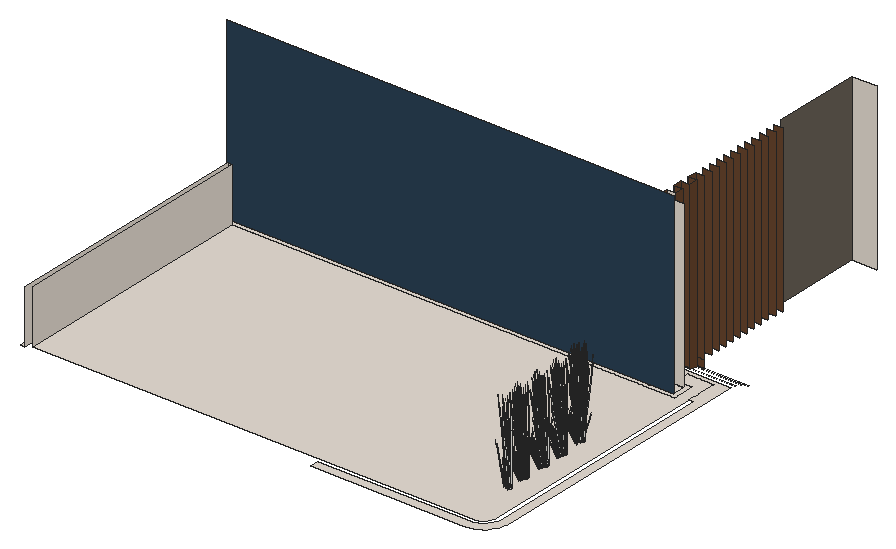
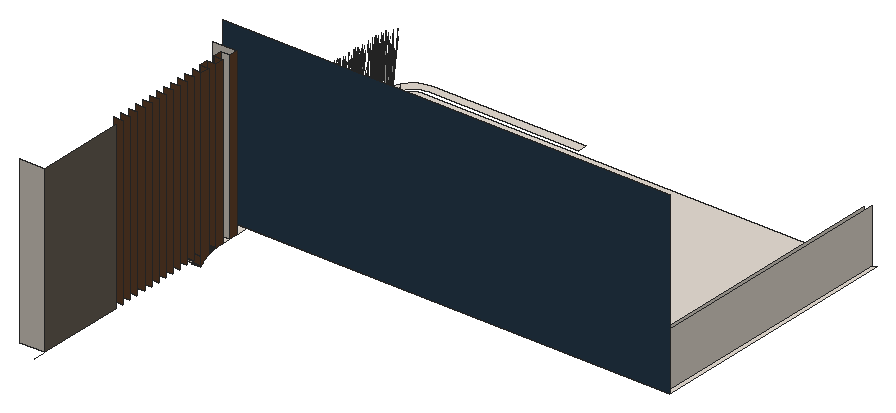
# SketchUp Ruby script. Lengths in inches.
U = 1.inch
M = Sketchup.active_model
def pt(a) = Geom::Point3d.new(a.map { |v| v * U })
def face(e, loops, mat)
  f = e.add_face(loops[0].map { |a| pt(a) })
  loops[1..].each { |l| e.add_face(l.map { |a| pt(a) }).erase! }
  f.material = f.back_material = mat if mat
  f
end
# faces: each face lists its corners as indices into pts; further lists are holes
def faces(e, pts, list, mat = nil) = list.each { |f| face(e, (f[0].is_a?(Array) ? f : [f]).map { |l| l.map { |i| pts[i] } }, mat) }
# xy, xz, yz: faces in a plane at the given z, y or x. An outline is a flat list of corners, or four numbers for a rectangle; further outlines are holes
def ring(l) = l.size == 4 ? [[l[0], l[1]], [l[2], l[1]], [l[2], l[3]], [l[0], l[3]]] : l.each_slice(2).to_a
def flat(e, list, mat, &to3) = list.each { |f| face(e, (f[0].is_a?(Array) ? f : [f]).map { |l| ring(l).map { |u, v| to3.(u, v) } }, mat) }
def xy(e, z, list, mat = nil) = flat(e, list, mat) { |x, y| [x, y, z] }
def xz(e, y, list, mat = nil) = flat(e, list, mat) { |x, z| [x, y, z] }
def yz(e, x, list, mat = nil) = flat(e, list, mat) { |y, z| [x, y, z] }
def lines(e, pts, list) = list.each { |a, b| e.add_line(pt(pts[a]), pt(pts[b])) }
# prism: a flat outline (further loops are holes) pulled along v
def prism(e, loops, v, mat = nil)
  f = face(e, loops, mat); d = Geom::Vector3d.new(v.map { |x| x * U })
  f.pushpull(f.normal.samedirection?(d) ? d.length : -d.length)
end
def box(e, o, s, mat = nil) = prism(e, [[o, [o[0] + s[0], o[1], o[2]], [o[0] + s[0], o[1] + s[1], o[2]], [o[0], o[1] + s[1], o[2]]]], [0, 0, s[2]], mat)
def at(x, y, z, deg = 0) = Geom::Transformation.translation(pt([x, y, z])) * Geom::Transformation.rotation(ORIGIN, Z_AXIS, deg.degrees)
def axes(o, x, y, z) = Geom::Transformation.new([*x, 0, *y, 0, *z, 0, *pt(o).to_a, 1])
def part(name) = M.definitions.add(name)
# library, detail: a bought-in or finely detailed component or shape, given as its bounding box
def library(name, o, s) = part(name).tap { |d| box(d.entities, o, s) }
def detail(e, o, s) = box(e.add_group.entities, o, s)
def put(e, d, t, mat = nil) = e.add_instance(d, t).tap { |i| i.material = mat if mat }
def group(e, t, mat = nil) = e.add_group.tap { |g| g.transformation = t; g.material = mat if mat }.entities
root = M.entities
M.materials.add("Carpet_04_1K").color = [43, 65, 85]
M.materials.add("LightPink_Translucent").color = [144, 107, 117]
M.materials["LightPink_Translucent"].alpha = 0.75
M.materials.add("Marble_01_1K").color = [230, 221, 211]
M.materials.add("Plaster_04_1K").color = [106, 98, 87]
M.materials.add("Wood_Veneer_15_1K").color = [103, 69, 45]
c1 = part("blade")
p = [[2.15,0.21,22],[0,0.17,0],[0.09,0.45,0],[2.18,0.31,22],[2.29,0.31,22],[0.38,0.45,0],
  [2.48,0.24,33],[2.49,0.24,33],[2.48,0.22,33]]
faces(c1.entities,p,[[0,1,2,3],[4,5,2,3],[6,3,4,7],[8,0,3,6]])
c2 = part("seeds")
p = [[0.3,-0.1,1.38],[-0.01,-0.03,1.59],[-0.01,-0.03,0.03],[0.14,-0.07,-0.07],[0.29,-0.03,3],[0.15,0.01,3.11]]
faces(c2.entities,p,[[0,1,2,3],[1,0,4,5]],"LightPink_Translucent")
c3 = part("blade with seeds")
put(c3.entities,c1,at(0,0,0))
put(c3.entities,c2,axes([2.4,0.25,30.99],[1.5799,-0.05474,1.17369],[-0.12525,1.92788,0.29478],[-0.07173,-0.02425,1.56792]))
xy(root,264,[[237,36,339,36,341.38,36.08,343.72,36.47,345.99,37.19,348.14,38.21,350.13,39.51,351.92,41.08,353.49,42.87,354.79,44.86,355.81,47.01,356.53,49.28,356.92,51.62,357,54,357,240,321,240,321,237,327,237,327,231,321,231,321,225,337.5,225,337.5,216,39,216,39,213,340.5,213,340.5,228,330,228,330,237,348,237,348,216,351,216,351,54,350.875,52.44,350.55,50.91,350.03,49.44,349.33,48.04,348.46,46.75,347.42,45.58,346.25,44.54,344.96,43.67,343.56,42.97,342.09,42.45,340.56,42.125,339,42,237,42],[36,42,39,216],[42,45,338.95,45,340.125,45.1,341.28,45.34,342.39,45.73,343.44,46.26,344.42,46.92,345.3,47.7,346.08,48.58,346.74,49.56,347.27,50.61,347.66,51.72,347.9,52.875,348,54.05,348,237,330,237,330,228,340.5,228,340.5,213,42,213],[321,216,337.5,225],[321,231,327,237]],"Marble_01_1K")
xz(root,213,[[39,264,42,300]],"Marble_01_1K")
xz(root,216,[[36,264,337.5,384]],"Carpet_04_1K")
xz(root,225,[[321,264,337.5,375]],"Marble_01_1K")
xz(root,231,[[321,264,327,375]],"Marble_01_1K")
xz(root,237,[[321,264,327,375]],"Wood_Veneer_15_1K")
xz(root,243,[[321,263.74,327,264]],"Marble_01_1K")
xz(root,243,[[321,264,327,375]],"Wood_Veneer_15_1K")
xz(root,249,[[321,262.04,327,264],[321,264,327,375]],"Wood_Veneer_15_1K")
xz(root,255,[[321,258.4,327,264],[321,264,327,375]],"Wood_Veneer_15_1K")
xz(root,261,[[321,264,327,375]],"Wood_Veneer_15_1K")
xz(root,267,[[321,264,327,375]],"Wood_Veneer_15_1K")
xz(root,273,[[321,264,327,375]],"Wood_Veneer_15_1K")
xz(root,279,[[321,264,327,375]],"Wood_Veneer_15_1K")
xz(root,285,[[321,264,327,375]],"Wood_Veneer_15_1K")
xz(root,291,[[321,264,327,375]],"Wood_Veneer_15_1K")
xz(root,297,[[321,264,327,375]],"Wood_Veneer_15_1K")
xz(root,303,[[321,264,327,375]],"Wood_Veneer_15_1K")
xz(root,309,[[321,264,327,375]],"Wood_Veneer_15_1K")
xz(root,315,[[321,264,327,375]],"Wood_Veneer_15_1K")
xz(root,321,[[321,264,327,375]],"Wood_Veneer_15_1K")
xz(root,387,[[321,264,337.5,375]],"Marble_01_1K")
yz(root,39,[[42,264,213,300]],"Marble_01_1K")
yz(root,42,[[45,264,213,300]],"Marble_01_1K")
yz(root,321,[[327,264,387,375]],"Plaster_04_1K")
yz(root,321,[[255,258.4,255,375,249,375,249,262.04,249.43,261.85,250.11,261.54,250.77,261.2,251.43,260.84,252.08,260.46,252.71,260.07,253.34,259.65,253.95,259.22,254.54,258.77],[242.98,263.74,243,263.74,243,375,237,375,237,264,240,264,240.75,263.97,241.49,263.91,242.24,263.84],[225,264,231,375]],"Wood_Veneer_15_1K")
yz(root,327,[[249,262.04,249,375,243,375,243,263.74,243.72,263.62,244.45,263.47,245.18,263.31,245.91,263.12,246.625,262.91,247.34,262.68,248.04,262.42,248.74,262.15],[231,264,237,375]],"Wood_Veneer_15_1K")
p = [[321,255.69,257.81],[321,255.125,258.3],[327,255.125,258.3],[327,255.69,257.81],[357,254.54,258.77],[357,255.125,258.3],
  [327,255,258.4],[321,255,258.4],[321,254.54,258.77],[357,248.74,262.15],[357,249.43,261.85],[321,249.43,261.85],
  [321,249,262.04],[327,249,262.04],[327,248.74,262.15],[321,248.74,262.15],[321,248.04,262.42],[327,248.04,262.42],
  [321,247.34,262.68],[327,247.34,262.68],[321,246.625,262.91],[327,246.625,262.91],[321,245.91,263.12],[327,245.91,263.12],
  [321,245.18,263.31],[327,245.18,263.31],[321,244.45,263.47],[327,244.45,263.47],[321,243.72,263.62],[327,243.72,263.62],
  [321,243,263.74],[327,243,263.74],[357,242.98,263.74],[357,243.72,263.62],[321,242.98,263.74],[321,387,264],
  [321,396,264]]
faces(root,p,[[0,1,2,3],[4,5,2,6,7,8],[1,7,6,2],[9,10,11,12,13,14],[12,15,14,13],[15,16,17,14],[16,18,19,17],[18,20,21,19],
  [20,22,23,21],[22,24,25,23],[24,26,27,25],[26,28,29,27],[28,30,31,29],[32,33,29,31,30,34]],"Marble_01_1K")
lines(root,p,[[35,36]])
put(root,c3,axes([330.66,143.87,266.41],[0.17773,0.04462,1.33163],[0.11455,0.45576,-0.28638],[-0.24142,0.08531,0.56934]))
put(root,c3,axes([331.35,141.67,266.41],[0.09985,0.15133,1.33163],[-0.23008,0.41134,-0.28638],[-0.23625,-0.09832,0.56934]))
put(root,c3,axes([330.99,142.68,265.39],[0.01297,0.08566,1.6421],[-0.26146,0.44735,-0.25086],[-0.18572,-0.02255,0.2797]))
put(root,c3,axes([330.85,145.08,265.39],[0.0686,0.0543,1.6421],[0.11632,0.50315,-0.25086],[-0.15204,0.10729,0.2797]))
put(root,c3,axes([332.875,125.86,266.41],[0.17773,0.04462,1.33163],[0.11455,0.45576,-0.28638],[-0.24142,0.08531,0.56934]))
put(root,c3,axes([332.875,110.02,266.41],[0.17773,0.04462,1.33163],[0.11455,0.45576,-0.28638],[-0.24142,0.08531,0.56934]))
put(root,c3,axes([332.875,93.61,266.41],[0.17773,0.04462,1.33163],[0.11455,0.45576,-0.28638],[-0.24142,0.08531,0.56934]))
put(root,c3,axes([332.875,78.72,266.41],[0.17773,0.04462,1.33163],[0.11455,0.45576,-0.28638],[-0.24142,0.08531,0.56934]))
put(root,c3,axes([332.7,143.46,265.92],[-0.53199,-0.08911,-0.58063],[0.11226,-0.54969,-0.15239],[-0.15876,-0.06661,1.28164]))
put(root,c3,axes([333.5625,123.66,266.41],[0.09985,0.15133,1.33163],[-0.23008,0.41134,-0.28638],[-0.23625,-0.09832,0.56934]))
put(root,c3,axes([333.5625,107.82,266.41],[0.09985,0.15133,1.33163],[-0.23008,0.41134,-0.28638],[-0.23625,-0.09832,0.56934]))
put(root,c3,axes([333.5625,91.4,266.41],[0.09985,0.15133,1.33163],[-0.23008,0.41134,-0.28638],[-0.23625,-0.09832,0.56934]))
put(root,c3,axes([332,144.5,265.88],[-0.47863,-0.27177,-0.46235],[0.28609,-0.48733,0],[-0.10901,-0.0619,1.46668]))
put(root,c3,axes([331.79,140.45,265.39],[-0.04954,0.0716,1.6421],[-0.50062,0.15438,-0.25086],[-0.12094,-0.14044,0.2797]))
put(root,c3,axes([332.29,144.83,266.21],[-0.31974,0.54466,0],[-0.53494,-0.30375,-0.48057],[-0.12184,-0.06918,1.52448]))
put(root,c3,axes([333.2,124.67,265.39],[0.01297,0.08566,1.6421],[-0.26146,0.44735,-0.25086],[-0.18572,-0.02255,0.2797]))
put(root,c3,axes([333.2,108.83,265.39],[0.01297,0.08566,1.6421],[-0.26146,0.44735,-0.25086],[-0.18572,-0.02255,0.2797]))
put(root,c3,axes([333.2,92.41,265.39],[0.01297,0.08566,1.6421],[-0.26146,0.44735,-0.25086],[-0.18572,-0.02255,0.2797]))
put(root,c3,axes([331.71,145.61,266.41],[0.16138,-0.08575,1.33163],[0.39845,0.25854,-0.28638],[-0.1186,0.22371,0.56934]))
put(root,c3,axes([331.48,140.73,265.98],[-0.14753,0.44383,-0.03625],[-0.45406,-0.13653,-0.16435],[-0.06894,-0.07259,0.54209]))
put(root,c3,axes([332.5,110.98,266.58],[0.21313,-0.24635,1.06958],[0.0841,0.38999,0.78586],[-0.15402,0.06983,0.23558]))
put(root,c3,axes([332.5,94.56,266.58],[0.21313,-0.24635,1.06958],[0.0841,0.38999,0.78586],[-0.15402,0.06983,0.23558]))
put(root,c3,axes([332.5,79.67,266.58],[0.21313,-0.24635,1.06958],[0.0841,0.38999,0.78586],[-0.15402,0.06983,0.23558]))
put(root,c3,axes([332.16,140.17,266.41],[-0.03097,0.17781,1.33163],[-0.45273,0.14885,-0.28638],[-0.10583,-0.22982,0.56934]))
put(root,c3,axes([333.3,143.54,266.48],[-0.51635,0.36087,-0.27094],[-0.34336,-0.5099,-0.46562],[-0.1274,-0.05178,1.4872]))
put(root,c3,axes([331.24,142.75,266.21],[-0.63949,0,0],[0,-0.60749,-0.48057],[0,-0.13836,1.52448]))
put(root,c3,axes([332.13,144.3,265.89],[-0.12013,-0.47362,-0.28847],[0.47712,-0.13449,0.28847],[-0.09619,-0.05462,1.29413]))
put(root,c3,axes([333.06,127.07,265.39],[0.0686,0.0543,1.6421],[0.11632,0.50315,-0.25086],[-0.15204,0.10729,0.2797]))
put(root,c3,axes([333.06,111.23,265.39],[0.0686,0.0543,1.6421],[0.11632,0.50315,-0.25086],[-0.15204,0.10729,0.2797]))
put(root,c3,axes([333.06,94.8125,265.39],[0.0686,0.0543,1.6421],[0.11632,0.50315,-0.25086],[-0.15204,0.10729,0.2797]))
put(root,c3,axes([333.06,79.93,265.39],[0.0686,0.0543,1.6421],[0.11632,0.50315,-0.25086],[-0.15204,0.10729,0.2797]))
put(root,c3,axes([332.97,124.11,266.58],[0.3265,-0.03889,1.06958],[-0.20711,0.3427,0.78586],[-0.16135,-0.05141,0.23558]))
put(root,c3,axes([332.97,108.27,266.58],[0.3265,-0.03889,1.06958],[-0.20711,0.3427,0.78586],[-0.16135,-0.05141,0.23558]))
put(root,c3,axes([332.97,91.85,266.58],[0.3265,-0.03889,1.06958],[-0.20711,0.3427,0.78586],[-0.16135,-0.05141,0.23558]))
put(root,c3,axes([333.65,143.93,265.92],[-0.34446,0.40855,-0.58063],[-0.42791,-0.37046,-0.15239],[-0.13803,0.10191,1.28164]))
put(root,c3,axes([331.73,142.59,266.17],[-0.47569,0.45698,0.2864],[-0.47598,-0.45217,-0.33981],[-0.01661,-0.12977,1.53541]))
put(root,c3,axes([333.88,143.7,266.3],[-0.49938,-0.43748,-0.23459],[0.42021,-0.49126,0.51337],[-0.13447,0.05118,1.56642]))
put(root,c3,axes([332.98,143.28,266.06],[-0.30722,-0.45622,-0.41661],[0.46535,-0.32126,0.2005],[-0.09942,-0.05645,1.33761]))
put(root,c3,axes([333.63,143.61,266.06],[-0.55535,0.03355,-0.41661],[-0.05022,-0.55698,0.2005],[-0.09942,0.05645,1.33761]))
put(root,c3,axes([332.57,144.54,266.31],[0.47863,0.27177,0.46235],[-0.28609,0.48733,0],[-0.10901,-0.0619,1.46668]))
put(root,c3,axes([334.91,125.45,265.92],[-0.53199,-0.08911,-0.58063],[0.11226,-0.54969,-0.15239],[-0.15876,-0.06661,1.28164]))
put(root,c3,axes([334.91,109.61,265.92],[-0.53199,-0.08911,-0.58063],[0.11226,-0.54969,-0.15239],[-0.15876,-0.06661,1.28164]))
put(root,c3,axes([334.92,93.19,265.92],[-0.53199,-0.08911,-0.58063],[0.11226,-0.54969,-0.15239],[-0.15876,-0.06661,1.28164]))
put(root,c3,axes([333.02,143.54,266.27],[0.13555,-0.64407,-0.21817],[0.64269,0.11227,0.47743],[-0.1123,-0.08895,1.45677]))
put(root,c3,axes([333.25,143.7,266.4375],[-0.09866,0.48509,0.13483],[-0.48202,-0.0842,-0.38503],[-0.08772,-0.04981,1.18024]))
put(root,c3,axes([334.21,145.05,265.88],[-0.47863,0.27177,-0.46235],[-0.28609,-0.48733,0],[-0.10901,0.0619,1.46668]))
put(root,c3,axes([331.38,142.34,265.88],[0,-0.54355,-0.46235],[0.57217,0,0],[0,-0.1238,1.46668]))
put(root,c3,axes([331.625,142.84,266.31],[0,0.54355,0.46235],[-0.57217,0,0],[0,-0.1238,1.46668]))
put(root,c3,axes([334.25,144.9,266.04],[-0.31576,-0.54657,-0.04789],[0.53494,-0.30375,0.48057],[-0.13182,0.05204,1.52373]))
put(root,c3,axes([334.22,126.49,265.88],[-0.47863,-0.27177,-0.46235],[0.28609,-0.48733,0],[-0.10901,-0.0619,1.46668]))
put(root,c3,axes([334.22,110.65,265.88],[-0.47863,-0.27177,-0.46235],[0.28609,-0.48733,0],[-0.10901,-0.0619,1.46668]))
put(root,c3,axes([334.22,94.23,265.88],[-0.47863,-0.27177,-0.46235],[0.28609,-0.48733,0],[-0.10901,-0.0619,1.46668]))
put(root,c3,axes([334.01,122.44,265.39],[-0.04954,0.0716,1.6421],[-0.50062,0.15438,-0.25086],[-0.12094,-0.14044,0.2797]))
put(root,c3,axes([334.01,106.6,265.39],[-0.04954,0.0716,1.6421],[-0.50062,0.15438,-0.25086],[-0.12094,-0.14044,0.2797]))
put(root,c3,axes([334.01,90.18,265.39],[-0.04954,0.0716,1.6421],[-0.50062,0.15438,-0.25086],[-0.12094,-0.14044,0.2797]))
put(root,c3,axes([334.1,144.83,265.89],[-0.47712,-0.13449,-0.28847],[0.12013,-0.47362,0.28847],[-0.09619,0.05462,1.29413]))
put(root,c3,axes([334.51,126.82,266.21],[-0.31974,0.54466,0],[-0.53494,-0.30375,-0.48057],[-0.12184,-0.06918,1.52448]))
put(root,c3,axes([334.51,110.98,266.21],[-0.31974,0.54466,0],[-0.53494,-0.30375,-0.48057],[-0.12184,-0.06918,1.52448]))
put(root,c3,axes([334.51,94.56,266.21],[-0.31974,0.54466,0],[-0.53494,-0.30375,-0.48057],[-0.12184,-0.06918,1.52448]))
put(root,c3,axes([334.51,79.67,266.21],[-0.31974,0.54466,0],[-0.53494,-0.30375,-0.48057],[-0.12184,-0.06918,1.52448]))
put(root,c3,axes([332.875,142.97,266.48],[-0.57594,-0.25935,-0.27094],[0.27732,-0.5474,-0.46562],[-0.0181,-0.1344,1.4872]))
put(root,c3,axes([331.82,145.2,266.63],[0.46459,-0.09625,0.0606],[0.10681,0.38778,-0.80367],[-0.02945,0.1963,0.72038]))
put(root,c3,axes([334.02,143.46,266.48],[0.05959,0.62022,-0.27094],[-0.62068,0.0375,-0.46562],[-0.1093,0.08261,1.4872]))
put(root,c3,axes([332.62,142.42,265.95],[-0.21003,-0.55738,-0.65031],[0.60499,-0.20074,-0.17068],[-0.02321,-0.18874,1.43544]))
put(root,c3,axes([333.93,127.61,266.41],[0.16138,-0.08575,1.33163],[0.39845,0.25854,-0.28638],[-0.1186,0.22371,0.56934]))
put(root,c3,axes([333.93,111.77,266.41],[0.16138,-0.08575,1.33163],[0.39845,0.25854,-0.28638],[-0.1186,0.22371,0.56934]))
put(root,c3,axes([333.93,95.35,266.41],[0.16138,-0.08575,1.33163],[0.39845,0.25854,-0.28638],[-0.1186,0.22371,0.56934]))
put(root,c3,axes([333.93,80.46,266.41],[0.16138,-0.08575,1.33163],[0.39845,0.25854,-0.28638],[-0.1186,0.22371,0.56934]))
put(root,c3,axes([333.7,122.72,265.98],[-0.14753,0.44383,-0.03625],[-0.45406,-0.13653,-0.16435],[-0.06894,-0.07259,0.54209]))
put(root,c3,axes([333.7,106.875,265.98],[-0.14753,0.44383,-0.03625],[-0.45406,-0.13653,-0.16435],[-0.06894,-0.07259,0.54209]))
put(root,c3,axes([333.7,90.46,265.98],[-0.14753,0.44383,-0.03625],[-0.45406,-0.13653,-0.16435],[-0.06894,-0.07259,0.54209]))
put(root,c3,axes([331.625,142.35,265.89],[0.35699,-0.33913,-0.28847],[0.35699,0.33913,0.28847],[0,-0.10923,1.29413]))
put(root,c3,axes([333.24,140.16,265.98],[-0.35341,0.31182,-0.03625],[-0.32382,-0.34152,-0.16435],[-0.0228,-0.09677,0.54209]))
put(root,c3,axes([333.09,143.23,266.2],[0.64638,0.11452,0.42607],[-0.13155,0.64678,0.16719],[-0.09446,-0.06245,1.47927]))
put(root,c3,axes([334.375,122.16,266.41],[-0.03097,0.17781,1.33163],[-0.45273,0.14885,-0.28638],[-0.10583,-0.22982,0.56934]))
put(root,c3,axes([334.375,106.32,266.41],[-0.03097,0.17781,1.33163],[-0.45273,0.14885,-0.28638],[-0.10583,-0.22982,0.56934]))
put(root,c3,axes([334.375,89.9,266.41],[-0.03097,0.17781,1.33163],[-0.45273,0.14885,-0.28638],[-0.10583,-0.22982,0.56934]))
put(root,c3,axes([335.52,125.53,266.48],[-0.51635,0.36087,-0.27094],[-0.34336,-0.5099,-0.46562],[-0.1274,-0.05178,1.4872]))
put(root,c3,axes([335.52,109.69,266.48],[-0.51635,0.36087,-0.27094],[-0.34336,-0.5099,-0.46562],[-0.1274,-0.05178,1.4872]))
put(root,c3,axes([335.52,93.27,266.48],[-0.51635,0.36087,-0.27094],[-0.34336,-0.5099,-0.46562],[-0.1274,-0.05178,1.4872]))
put(root,c3,axes([332.93,143.12,266.53],[-0.24813,0.48978,0.41661],[-0.51557,-0.23571,-0.2005],[0,-0.1129,1.33761]))
put(root,c3,axes([333.45,124.74,266.21],[-0.63949,0,0],[0,-0.60749,-0.48057],[0,-0.13836,1.52448]))
put(root,c3,axes([333.45,108.9,266.21],[-0.63949,0,0],[0,-0.60749,-0.48057],[0,-0.13836,1.52448]))
put(root,c3,axes([333.45,92.48,266.21],[-0.63949,0,0],[0,-0.60749,-0.48057],[0,-0.13836,1.52448]))
put(root,c3,axes([334.35,126.29,265.89],[-0.12013,-0.47362,-0.28847],[0.47712,-0.13449,0.28847],[-0.09619,-0.05462,1.29413]))
put(root,c3,axes([334.35,110.45,265.89],[-0.12013,-0.47362,-0.28847],[0.47712,-0.13449,0.28847],[-0.09619,-0.05462,1.29413]))
put(root,c3,axes([334.35,94.03,265.89],[-0.12013,-0.47362,-0.28847],[0.47712,-0.13449,0.28847],[-0.09619,-0.05462,1.29413]))
put(root,c3,axes([332.75,144.27,266.3],[0.54955,-0.14427,0.16428],[0.1357,0.53689,0.32672],[-0.04901,-0.07823,1.49371]))
put(root,c3,axes([333.45,144.35,266.05],[-0.51557,-0.24403,0],[0.24813,-0.50705,0],[0,0,1.51513]))
put(root,c3,axes([335.86,125.92,265.92],[-0.34446,0.40855,-0.58063],[-0.42791,-0.37046,-0.15239],[-0.13803,0.10191,1.28164]))
put(root,c3,axes([335.86,110.08,265.92],[-0.34446,0.40855,-0.58063],[-0.42791,-0.37046,-0.15239],[-0.13803,0.10191,1.28164]))
put(root,c3,axes([335.86,93.67,265.92],[-0.34446,0.40855,-0.58063],[-0.42791,-0.37046,-0.15239],[-0.13803,0.10191,1.28164]))
put(root,c3,axes([335.86,78.78,265.92],[-0.34446,0.40855,-0.58063],[-0.42791,-0.37046,-0.15239],[-0.13803,0.10191,1.28164]))
put(root,c3,axes([334.65,144.96,266.21],[0.31974,0.54466,0],[-0.53494,0.30375,-0.48057],[-0.12184,0.06918,1.52448]))
put(root,c3,axes([333.95,124.58,266.17],[-0.47569,0.45698,0.2864],[-0.47598,-0.45217,-0.33981],[-0.01661,-0.12977,1.53541]))
put(root,c3,axes([333.95,108.74,266.17],[-0.47569,0.45698,0.2864],[-0.47598,-0.45217,-0.33981],[-0.01661,-0.12977,1.53541]))
put(root,c3,axes([333.95,92.32,266.17],[-0.47569,0.45698,0.2864],[-0.47598,-0.45217,-0.33981],[-0.01661,-0.12977,1.53541]))
put(root,c3,axes([334.38,144.3,266.3],[0.14774,-0.54019,0.16428],[0.54062,0.15287,0.32672],[-0.09339,0.00263,1.49371]))
put(root,c3,axes([334.22,106.03,266.58],[0.26677,0.18918,1.06958],[-0.38851,0.11372,0.78586],[-0.08313,-0.14539,0.23558]))
put(root,c3,axes([334.22,89.61,266.58],[0.26677,0.18918,1.06958],[-0.38851,0.11372,0.78586],[-0.08313,-0.14539,0.23558]))
put(root,c3,axes([334.13,143.58,266.4375],[0.37783,0.32657,0.13483],[-0.31516,0.36844,-0.38503],[-0.08772,0.04981,1.18024]))
put(root,c3,axes([336.1,125.69,266.3],[-0.49938,-0.43748,-0.23459],[0.42021,-0.49126,0.51337],[-0.13447,0.05118,1.56642]))
put(root,c3,axes([336.1,109.85,266.3],[-0.49938,-0.43748,-0.23459],[0.42021,-0.49126,0.51337],[-0.13447,0.05118,1.56642]))
put(root,c3,axes([336.1,93.4375,266.3],[-0.49938,-0.43748,-0.23459],[0.42021,-0.49126,0.51337],[-0.13447,0.05118,1.56642]))
put(root,c3,axes([335.19,125.27,266.06],[-0.30722,-0.45622,-0.41661],[0.46535,-0.32126,0.2005],[-0.09942,-0.05645,1.33761]))
put(root,c3,axes([335.19,109.43,266.06],[-0.30722,-0.45622,-0.41661],[0.46535,-0.32126,0.2005],[-0.09942,-0.05645,1.33761]))
put(root,c3,axes([335.19,93.02,266.06],[-0.30722,-0.45622,-0.41661],[0.46535,-0.32126,0.2005],[-0.09942,-0.05645,1.33761]))
put(root,c3,axes([334,143.18,266.14],[-0.47569,-0.46784,-0.05709],[0.47598,-0.46812,0],[-0.01661,-0.01634,1.63492]))
put(root,c3,axes([334.125,143.34,266.53],[0.55535,-0.03355,0.41661],[0.05022,0.55698,-0.2005],[-0.09942,0.05645,1.33761]))
put(root,c3,axes([334.3125,112.05,266.58],[-0.01324,-0.32319,1.06958],[0.33072,0.23052,0.78586],[-0.06504,0.15405,0.23558]))
put(root,c3,axes([334.3125,95.63,266.58],[-0.01324,-0.32319,1.06958],[0.33072,0.23052,0.78586],[-0.06504,0.15405,0.23558]))
put(root,c3,axes([334.3125,80.75,266.58],[-0.01324,-0.32319,1.06958],[0.33072,0.23052,0.78586],[-0.06504,0.15405,0.23558]))
put(root,c3,axes([334.26,144.62,266.17],[0.64025,0.17667,0.2864],[-0.16018,0.63149,-0.33981],[-0.10597,0.07904,1.53541]))
put(root,c3,axes([335.85,125.6,266.06],[-0.55535,0.03355,-0.41661],[-0.05022,-0.55698,0.2005],[-0.09942,0.05645,1.33761]))
put(root,c3,axes([335.85,109.76,266.06],[-0.55535,0.03355,-0.41661],[-0.05022,-0.55698,0.2005],[-0.09942,0.05645,1.33761]))
put(root,c3,axes([335.85,93.34,266.06],[-0.55535,0.03355,-0.41661],[-0.05022,-0.55698,0.2005],[-0.09942,0.05645,1.33761]))
put(root,c3,axes([335.85,78.46,266.06],[-0.55535,0.03355,-0.41661],[-0.05022,-0.55698,0.2005],[-0.09942,0.05645,1.33761]))
put(root,c3,axes([333.33,139.78,265.39],[-0.08578,0.01958,1.6421],[-0.47437,-0.22044,-0.25086],[0.00796,-0.18387,0.2797]))
put(root,c3,axes([334.54,144.59,266.31],[0.47863,-0.27177,0.46235],[0.28609,0.48733,0],[-0.10901,0.0619,1.46668]))
put(root,c3,axes([333.04,142.64,266.2],[0.22235,0.6078,0.42607],[-0.63531,0.21135,0.16719],[0.00776,-0.11168,1.47927]))
put(root,c3,axes([332.9375,142.5625,266.06],[0.24813,-0.48978,-0.41661],[0.51557,0.23571,0.2005],[0,-0.1129,1.33761]))
put(root,c3,axes([333.57,144.14,266.05],[-0.16686,-0.46861,0],[0.47648,-0.16411,0],[0,0,1.4375]))
put(root,c3,axes([334.78,126.53,266.31],[0.47863,0.27177,0.46235],[-0.28609,0.48733,0],[-0.10901,-0.0619,1.46668]))
put(root,c3,axes([334.78,110.69,266.31],[0.47863,0.27177,0.46235],[-0.28609,0.48733,0],[-0.10901,-0.0619,1.46668]))
put(root,c3,axes([334.78,94.27,266.31],[0.47863,0.27177,0.46235],[-0.28609,0.48733,0],[-0.10901,-0.0619,1.46668]))
put(root,c3,axes([332.97,145.13,265.39],[0.08277,-0.02958,1.6421],[0.49786,0.16279,-0.25086],[0.01456,0.18348,0.2797]))
put(root,c3,axes([335.24,125.53,266.27],[0.13555,-0.64407,-0.21817],[0.64269,0.11227,0.47743],[-0.1123,-0.08895,1.45677]))
put(root,c3,axes([335.24,109.7,266.27],[0.13555,-0.64407,-0.21817],[0.64269,0.11227,0.47743],[-0.1123,-0.08895,1.45677]))
put(root,c3,axes([335.24,93.28,266.27],[0.13555,-0.64407,-0.21817],[0.64269,0.11227,0.47743],[-0.1123,-0.08895,1.45677]))
put(root,c3,axes([335.47,125.6875,266.4375],[-0.09866,0.48509,0.13483],[-0.48202,-0.0842,-0.38503],[-0.08772,-0.04981,1.18024]))
put(root,c3,axes([335.47,109.85,266.4375],[-0.09866,0.48509,0.13483],[-0.48202,-0.0842,-0.38503],[-0.08772,-0.04981,1.18024]))
put(root,c3,axes([335.47,93.43,266.4375],[-0.09866,0.48509,0.13483],[-0.48202,-0.0842,-0.38503],[-0.08772,-0.04981,1.18024]))
put(root,c3,axes([336.43,127.04,265.88],[-0.47863,0.27177,-0.46235],[-0.28609,-0.48733,0],[-0.10901,0.0619,1.46668]))
put(root,c3,axes([336.43,111.2,265.88],[-0.47863,0.27177,-0.46235],[-0.28609,-0.48733,0],[-0.10901,0.0619,1.46668]))
put(root,c3,axes([336.43,94.78,265.88],[-0.47863,0.27177,-0.46235],[-0.28609,-0.48733,0],[-0.10901,0.0619,1.46668]))
put(root,c3,axes([336.43,79.89,265.88],[-0.47863,0.27177,-0.46235],[-0.28609,-0.48733,0],[-0.10901,0.0619,1.46668]))
put(root,c3,axes([333.6,124.33,265.88],[0,-0.54355,-0.46235],[0.57217,0,0],[0,-0.1238,1.46668]))
put(root,c3,axes([333.6,108.49,265.88],[0,-0.54355,-0.46235],[0.57217,0,0],[0,-0.1238,1.46668]))
put(root,c3,axes([333.6,92.07,265.88],[0,-0.54355,-0.46235],[0.57217,0,0],[0,-0.1238,1.46668]))
put(root,c3,axes([333.84,124.83,266.31],[0,0.54355,0.46235],[-0.57217,0,0],[0,-0.1238,1.46668]))
put(root,c3,axes([333.84,109,266.31],[0,0.54355,0.46235],[-0.57217,0,0],[0,-0.1238,1.46668]))
put(root,c3,axes([333.84,92.58,266.31],[0,0.54355,0.46235],[-0.57217,0,0],[0,-0.1238,1.46668]))
put(root,c3,axes([336.46,126.89,266.04],[-0.31576,-0.54657,-0.04789],[0.53494,-0.30375,0.48057],[-0.13182,0.05204,1.52373]))
put(root,c3,axes([336.46,111.05,266.04],[-0.31576,-0.54657,-0.04789],[0.53494,-0.30375,0.48057],[-0.13182,0.05204,1.52373]))
put(root,c3,axes([336.46,94.63,266.04],[-0.31576,-0.54657,-0.04789],[0.53494,-0.30375,0.48057],[-0.13182,0.05204,1.52373]))
put(root,c3,axes([336.46,79.75,266.04],[-0.31576,-0.54657,-0.04789],[0.53494,-0.30375,0.48057],[-0.13182,0.05204,1.52373]))
put(root,c3,axes([334.25,143.22,266.06],[-0.24813,0.48978,-0.41661],[-0.51557,-0.23571,0.2005],[0,0.1129,1.33761]))
put(root,c3,axes([336.32,126.82,265.89],[-0.47712,-0.13449,-0.28847],[0.12013,-0.47362,0.28847],[-0.09619,0.05462,1.29413]))
put(root,c3,axes([336.32,110.98,265.89],[-0.47712,-0.13449,-0.28847],[0.12013,-0.47362,0.28847],[-0.09619,0.05462,1.29413]))
put(root,c3,axes([336.32,94.57,265.89],[-0.47712,-0.13449,-0.28847],[0.12013,-0.47362,0.28847],[-0.09619,0.05462,1.29413]))
put(root,c3,axes([336.32,79.68,265.89],[-0.47712,-0.13449,-0.28847],[0.12013,-0.47362,0.28847],[-0.09619,0.05462,1.29413]))
put(root,c3,axes([335.23,142.92,266.3],[-0.40181,-0.39593,0.16428],[0.40492,-0.38402,0.32672],[-0.04438,0.08086,1.49371]))
put(root,c3,axes([333.84,142.69,266.05],[0,-0.62892,0],[0.63949,0,0],[0,0,1.6711]))
put(root,c3,axes([335.09,124.96,266.48],[-0.57594,-0.25935,-0.27094],[0.27732,-0.5474,-0.46562],[-0.0181,-0.1344,1.4872]))
put(root,c3,axes([335.09,109.12,266.48],[-0.57594,-0.25935,-0.27094],[0.27732,-0.5474,-0.46562],[-0.0181,-0.1344,1.4872]))
put(root,c3,axes([335.09,92.7,266.48],[-0.57594,-0.25935,-0.27094],[0.27732,-0.5474,-0.46562],[-0.0181,-0.1344,1.4872]))
put(root,c3,axes([333.24,142.8,266.27],[0.57623,0.26344,0.22409],[-0.27732,0.5474,0.46562],[0,-0.12618,1.49497]))
put(root,c3,axes([334.16,142.94,266.13],[0,0.62861,-0.05249],[-0.63949,0,0],[0,0.01975,1.67027]))
put(root,c3,axes([333.06,142.4375,266.53],[-0.55535,0.03355,0.41661],[-0.05022,-0.55698,-0.2005],[0.09942,-0.05645,1.33761]))
put(root,c3,axes([332.8,141.48,266.3],[-0.14774,0.54019,0.16428],[-0.54062,-0.15287,0.32672],[0.09339,-0.00263,1.49371]))
put(root,c3,axes([333.85,144.16,266.13],[0.22235,0.62444,-0.05599],[-0.63531,0.21881,0],[0.00776,0.02181,1.60327]))
put(root,c3,axes([334.04,127.19,266.63],[0.46459,-0.09625,0.0606],[0.10681,0.38778,-0.80367],[-0.02945,0.1963,0.72038]))
put(root,c3,axes([334.04,111.35,266.63],[0.46459,-0.09625,0.0606],[0.10681,0.38778,-0.80367],[-0.02945,0.1963,0.72038]))
put(root,c3,axes([334.04,94.9375,266.63],[0.46459,-0.09625,0.0606],[0.10681,0.38778,-0.80367],[-0.02945,0.1963,0.72038]))
put(root,c3,axes([334.04,80.05,266.63],[0.46459,-0.09625,0.0606],[0.10681,0.38778,-0.80367],[-0.02945,0.1963,0.72038]))
put(root,c3,axes([336.23,125.45,266.48],[0.05959,0.62022,-0.27094],[-0.62068,0.0375,-0.46562],[-0.1093,0.08261,1.4872]))
put(root,c3,axes([336.23,109.61,266.48],[0.05959,0.62022,-0.27094],[-0.62068,0.0375,-0.46562],[-0.1093,0.08261,1.4872]))
put(root,c3,axes([336.23,93.19,266.48],[0.05959,0.62022,-0.27094],[-0.62068,0.0375,-0.46562],[-0.1093,0.08261,1.4872]))
put(root,c3,axes([336.23,78.31,266.48],[0.05959,0.62022,-0.27094],[-0.62068,0.0375,-0.46562],[-0.1093,0.08261,1.4872]))
put(root,c3,axes([334.83,124.41,265.95],[-0.21003,-0.55738,-0.65031],[0.60499,-0.20074,-0.17068],[-0.02321,-0.18874,1.43544]))
put(root,c3,axes([334.83,108.57,265.95],[-0.21003,-0.55738,-0.65031],[0.60499,-0.20074,-0.17068],[-0.02321,-0.18874,1.43544]))
put(root,c3,axes([334.83,92.15,265.95],[-0.21003,-0.55738,-0.65031],[0.60499,-0.20074,-0.17068],[-0.02321,-0.18874,1.43544]))
put(root,c3,axes([332.53,140.81,266.21],[-0.31974,-0.54466,0],[0.53494,-0.30375,-0.48057],[0.12184,-0.06918,1.52448]))
put(root,c3,axes([335.69,143.34,266.05],[-0.63917,-0.00435,-0.04634],[0,-0.60749,0.46507],[-0.02009,0.13829,1.47457]))
put(root,c3,axes([333.84,124.34,265.89],[0.35699,-0.33913,-0.28847],[0.35699,0.33913,0.28847],[0,-0.10923,1.29413]))
put(root,c3,axes([333.84,108.5,265.89],[0.35699,-0.33913,-0.28847],[0.35699,0.33913,0.28847],[0,-0.10923,1.29413]))
put(root,c3,axes([333.84,92.08,265.89],[0.35699,-0.33913,-0.28847],[0.35699,0.33913,0.28847],[0,-0.10923,1.29413]))
put(root,c3,axes([335.45,122.15,265.98],[-0.35341,0.31182,-0.03625],[-0.32382,-0.34152,-0.16435],[-0.0228,-0.09677,0.54209]))
put(root,c3,axes([335.45,106.31,265.98],[-0.35341,0.31182,-0.03625],[-0.32382,-0.34152,-0.16435],[-0.0228,-0.09677,0.54209]))
put(root,c3,axes([335.45,89.89,265.98],[-0.35341,0.31182,-0.03625],[-0.32382,-0.34152,-0.16435],[-0.0228,-0.09677,0.54209]))
put(root,c3,axes([334.43,141.51,266.3],[-0.54955,0.14427,0.16428],[-0.1357,-0.53689,0.32672],[0.04901,0.07823,1.49371]))
put(root,c3,axes([335.31,125.22,266.2],[0.64638,0.11452,0.42607],[-0.13155,0.64678,0.16719],[-0.09446,-0.06245,1.47927]))
put(root,c3,axes([335.31,109.39,266.2],[0.64638,0.11452,0.42607],[-0.13155,0.64678,0.16719],[-0.09446,-0.06245,1.47927]))
put(root,c3,axes([335.31,92.97,266.2],[0.64638,0.11452,0.42607],[-0.13155,0.64678,0.16719],[-0.09446,-0.06245,1.47927]))
put(root,c3,axes([333.54,142.29,266.2],[-0.42403,0.49328,0.42607],[-0.50377,-0.43543,0.16719],[0.10223,-0.04923,1.47927]))
put(root,c3,axes([335.14,125.11,266.53],[-0.24813,0.48978,0.41661],[-0.51557,-0.23571,-0.2005],[0,-0.1129,1.33761]))
put(root,c3,axes([335.14,109.27,266.53],[-0.24813,0.48978,0.41661],[-0.51557,-0.23571,-0.2005],[0,-0.1129,1.33761]))
put(root,c3,axes([335.14,92.85,266.53],[-0.24813,0.48978,0.41661],[-0.51557,-0.23571,-0.2005],[0,-0.1129,1.33761]))
put(root,c3,axes([334.26,143.07,266.0625],[0.35699,0.35109,0],[-0.35699,0.35109,0],[0,0,1.57621]))
put(root,c3,axes([334.26,142.66,266.53],[0.24813,-0.48978,0.41661],[0.51557,0.23571,-0.2005],[0,0.1129,1.33761]))
put(root,c3,axes([334.04,144.36,266.05],[0.51557,0.24403,0],[-0.24813,0.50705,0],[0,0,1.62917]))
put(root,c3,axes([334.09,142.54,266.22],[-0.64638,-0.11452,0.45814],[0.13155,-0.64678,0.17978],[0.09446,0.06245,1.59061]))
put(root,c3,axes([334.96,126.26,266.3],[0.54955,-0.14427,0.16428],[0.1357,0.53689,0.32672],[-0.04901,-0.07823,1.49371]))
put(root,c3,axes([334.96,110.42,266.3],[0.54955,-0.14427,0.16428],[0.1357,0.53689,0.32672],[-0.04901,-0.07823,1.49371]))
put(root,c3,axes([334.96,94,266.3],[0.54955,-0.14427,0.16428],[0.1357,0.53689,0.32672],[-0.04901,-0.07823,1.49371]))
put(root,c3,axes([335.56,143.43,265.89],[-0.35699,0.33913,-0.28847],[-0.35699,-0.33913,0.28847],[0,0.10923,1.29413]))
put(root,c3,axes([335.67,126.34,266.05],[-0.51557,-0.24403,0],[0.24813,-0.50705,0],[0,0,1.51513]))
put(root,c3,axes([335.67,110.5,266.05],[-0.51557,-0.24403,0],[0.24813,-0.50705,0],[0,0,1.51513]))
put(root,c3,axes([335.67,94.09,266.05],[-0.51557,-0.24403,0],[0.24813,-0.50705,0],[0,0,1.51513]))
put(root,c3,axes([336.86,126.95,266.21],[0.31974,0.54466,0],[-0.53494,0.30375,-0.48057],[-0.12184,0.06918,1.52448]))
put(root,c3,axes([336.86,111.11,266.21],[0.31974,0.54466,0],[-0.53494,0.30375,-0.48057],[-0.12184,0.06918,1.52448]))
put(root,c3,axes([336.86,94.7,266.21],[0.31974,0.54466,0],[-0.53494,0.30375,-0.48057],[-0.12184,0.06918,1.52448]))
put(root,c3,axes([336.86,79.81,266.21],[0.31974,0.54466,0],[-0.53494,0.30375,-0.48057],[-0.12184,0.06918,1.52448]))
put(root,c3,axes([334.54,143.36,265.95],[0.18752,0.49766,-0.6445],[-0.54017,0.17923,-0.16915],[0.02073,0.16852,1.42262]))
put(root,c3,axes([334.27,142.83,266.05],[0.57217,0,0],[0,0.56272,0],[0,0,1.66132]))
put(root,c3,axes([333.72,142.21,266.53],[-0.30722,-0.45622,0.41661],[0.46535,-0.32126,-0.2005],[0.09942,0.05645,1.33761]))
put(root,c3,axes([333.16,142.32,266.48],[-0.05959,-0.62022,-0.27094],[0.62068,-0.0375,-0.46562],[0.1093,-0.08261,1.4872]))
put(root,c3,axes([334.47,142.77,266.4375],[0.47648,-0.15851,0.13483],[0.16686,0.45265,-0.38503],[0,0.09962,1.18024]))
put(root,c3,axes([336.6,126.29,266.3],[0.14774,-0.54019,0.16428],[0.54062,0.15287,0.32672],[-0.09339,0.00263,1.49371]))
put(root,c3,axes([336.6,110.45,266.3],[0.14774,-0.54019,0.16428],[0.54062,0.15287,0.32672],[-0.09339,0.00263,1.49371]))
put(root,c3,axes([336.6,94.03,266.3],[0.14774,-0.54019,0.16428],[0.54062,0.15287,0.32672],[-0.09339,0.00263,1.49371]))
put(root,c3,axes([336.35,125.57,266.4375],[0.37783,0.32657,0.13483],[-0.31516,0.36844,-0.38503],[-0.08772,0.04981,1.18024]))
